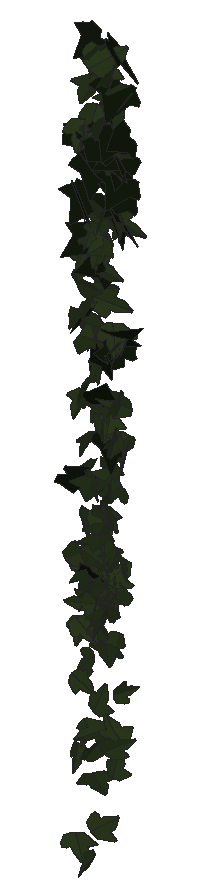
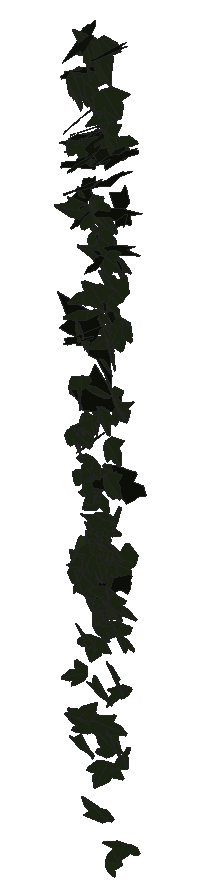
# SketchUp Ruby script. Lengths in inches.
U = 1.inch
M = Sketchup.active_model
def pt(a) = Geom::Point3d.new(a.map { |v| v * U })
def face(e, loops, mat)
  f = e.add_face(loops[0].map { |a| pt(a) })
  loops[1..].each { |l| e.add_face(l.map { |a| pt(a) }).erase! }
  f.material = f.back_material = mat if mat
  f
end
# faces: each face lists its corners as indices into pts; further lists are holes
def faces(e, pts, list, mat = nil) = list.each { |f| face(e, (f[0].is_a?(Array) ? f : [f]).map { |l| l.map { |i| pts[i] } }, mat) }
# xy, xz, yz: faces in a plane at the given z, y or x. An outline is a flat list of corners, or four numbers for a rectangle; further outlines are holes
def ring(l) = l.size == 4 ? [[l[0], l[1]], [l[2], l[1]], [l[2], l[3]], [l[0], l[3]]] : l.each_slice(2).to_a
def flat(e, list, mat, &to3) = list.each { |f| face(e, (f[0].is_a?(Array) ? f : [f]).map { |l| ring(l).map { |u, v| to3.(u, v) } }, mat) }
def xy(e, z, list, mat = nil) = flat(e, list, mat) { |x, y| [x, y, z] }
def xz(e, y, list, mat = nil) = flat(e, list, mat) { |x, z| [x, y, z] }
def yz(e, x, list, mat = nil) = flat(e, list, mat) { |y, z| [x, y, z] }
def lines(e, pts, list) = list.each { |a, b| e.add_line(pt(pts[a]), pt(pts[b])) }
# prism: a flat outline (further loops are holes) pulled along v
def prism(e, loops, v, mat = nil)
  f = face(e, loops, mat); d = Geom::Vector3d.new(v.map { |x| x * U })
  f.pushpull(f.normal.samedirection?(d) ? d.length : -d.length)
end
def box(e, o, s, mat = nil) = prism(e, [[o, [o[0] + s[0], o[1], o[2]], [o[0] + s[0], o[1] + s[1], o[2]], [o[0], o[1] + s[1], o[2]]]], [0, 0, s[2]], mat)
def at(x, y, z, deg = 0) = Geom::Transformation.translation(pt([x, y, z])) * Geom::Transformation.rotation(ORIGIN, Z_AXIS, deg.degrees)
def axes(o, x, y, z) = Geom::Transformation.new([*x, 0, *y, 0, *z, 0, *pt(o).to_a, 1])
def part(name) = M.definitions.add(name)
# library, detail: a bought-in or finely detailed component or shape, given as its bounding box
def library(name, o, s) = part(name).tap { |d| box(d.entities, o, s) }
def detail(e, o, s) = box(e.add_group.entities, o, s)
def put(e, d, t, mat = nil) = e.add_instance(d, t).tap { |i| i.material = mat if mat }
def group(e, t, mat = nil) = e.add_group.tap { |g| g.transformation = t; g.material = mat if mat }.entities
root = M.entities
M.materials.add("1026 AP 7946 SUNNY SIDE UP").color = [254, 231, 186]
M.materials.add("efeu1").color = [18, 25, 13]
M.materials.add("efeu2").color = [43, 57, 29]
c1 = part("ivyleaf_10")
p = [[0,0.5,-0.03],[-0.0625,2.02,-0.43],[-0.19,2.01,-0.46],[-0.54,1.05,-0.29],[-0.52,0.625,-0.18],[-0.83,0.76,-0.28],
  [-1.16,0.64,-0.33],[-1.15,0.33,-0.24],[-0.77,-0.39,0.02],[-0.3,-0.51,0.16],[0.04,-0.48,0.23],[-0.02,2.01,-0.4375],
  [-0.06,2.01,-0.43],[0.04,-0.49,0.23],[0.67,-0.49,0.14],[1.38,0.36,-0.2],[1.375,0.51,-0.24],[0.81,0.65,-0.19],
  [0.62,0.59,-0.15],[0.6,1.09,-0.28],[0.5,1.23,-0.31]]
faces(c1.entities,p,[[0,1,2,3,4,5,6,7,8,9,10],[11,12,0,13,14,15,16,17,18,19,20]],"efeu2")
c2 = part("ivyleaf_9")
p = [[1.54,2.16,1.25],[1.36,2.04,1.19],[-0.21,0.99,0.68],[-0.71,1.11,0.82],[-0.85,0.86,0.67],[-0.8,0.17,0.21],
  [-0.9,-0.01,0.1],[-0.67,-0.16,-0.02],[-0.08,-0.08,-0.05],[-0.03,-0.6,-0.4],[0.65,-0.88,-0.66],[0.83,-0.6,-0.49],
  [1.29,-0.42,-0.43],[1.8125,-0.07,-0.26],[1.21,0.44,0.15]]
faces(c2.entities,p,[[0,1,2,3,4,5,6,7,8,9,10,11,12,13,14]],"efeu1")
put(root,c1,axes([102.35,212.49,259.8],[-0.06688,-0.16371,0.15021],[0.07926,-0.15273,-0.16139],[0.33648,0.00344,0.06787]),"1026 AP 7946 SUNNY SIDE UP")
put(root,c2,axes([102.26,212.62,265.65],[-0.01705,-0.2455,-0.06618],[0.02244,0.06221,-0.25253],[0.39784,-0.01403,0.01141]),"1026 AP 7946 SUNNY SIDE UP")
put(root,c1,axes([102.35,212.43,261.7],[-0.06038,-0.19316,-0.16336],[0.10843,0.14488,-0.19955],[0.37656,-0.07269,0.03126]),"1026 AP 7946 SUNNY SIDE UP")
put(root,c1,axes([102.32,212.39,253.47],[0.05045,0.17084,0.12661],[0.05043,0.11791,-0.1782],[-0.32616,0.04466,-0.00797]),"1026 AP 7946 SUNNY SIDE UP")
put(root,c2,axes([102.45,212.63,264.3125],[-0.27752,-0.16463,0.01399],[0.00167,-0.02237,-0.24815],[0.25986,-0.17567,0.01654]),"1026 AP 7946 SUNNY SIDE UP")
put(root,c1,axes([102.34,212.45,254.69],[0.29099,-0.088,0.05389],[0.06145,-0.04027,-0.21044],[0.14922,0.18819,-0.01844]),"1026 AP 7946 SUNNY SIDE UP")
put(root,c1,axes([102.39,212.5,265.87],[0.29429,0.15936,-0.05989],[-0.04948,-0.05381,-0.25271],[-0.26261,0.18873,-0.0195]),"1026 AP 7946 SUNNY SIDE UP")
put(root,c1,axes([102.39,212.33,251.92],[0.03154,0.19338,-0.12033],[-0.03166,-0.11637,-0.20084],[-0.35472,0.02758,0.00722]),"1026 AP 7946 SUNNY SIDE UP")
put(root,c1,axes([102.47,212.65,258.25],[0.00646,-0.19667,0.0764],[-0.00698,-0.07536,-0.20301],[0.33105,0.00225,-0.00577]),"1026 AP 7946 SUNNY SIDE UP")
put(root,c1,axes([102.46,212.47,260.07],[0.11644,-0.22452,0.02799],[0.0032,-0.02926,-0.24361],[0.35584,0.07373,-0.00696]),"1026 AP 7946 SUNNY SIDE UP")
put(root,c1,axes([102.52,212.53,253.93],[0.18226,-0.16859,-0.09209],[-0.09963,0.06347,-0.20983],[0.28228,0.13125,-0.0146]),"1026 AP 7946 SUNNY SIDE UP")
put(root,c1,axes([102.54,212.65,266.89],[-0.18408,-0.19871,0.10836],[-0.03233,-0.10989,-0.23556],[0.35289,-0.11373,0.03495]),"1026 AP 7946 SUNNY SIDE UP")
put(root,c1,axes([102.47,212.64,263.22],[-0.01801,-0.16096,0.17874],[0.05034,-0.17407,-0.16434],[0.36977,0.01586,0.03108]),"1026 AP 7946 SUNNY SIDE UP")
put(root,c2,axes([102.58,212.61,263.4],[-0.28153,-0.13286,0.10644],[-0.101,-0.08667,-0.22833],[0.24541,-0.18809,0.02814]),"1026 AP 7946 SUNNY SIDE UP")
put(root,c1,axes([102.35,212.23,256.3],[-0.06701,-0.08618,0.22956],[0.11622,0.21101,0.09965],[-0.358,0.08463,-0.01062]),"1026 AP 7946 SUNNY SIDE UP")
put(root,c1,axes([102.36,212.31,249.9],[0.27831,0.09746,0.05304],[0.08373,0.00848,-0.2073],[-0.15129,0.18398,-0.01716]),"1026 AP 7946 SUNNY SIDE UP")
put(root,c1,axes([102.49,212.57,255.39],[0.04011,-0.18599,0.09118],[0.01307,-0.08925,-0.19389],[0.32434,0.02659,-0.00347]),"1026 AP 7946 SUNNY SIDE UP")
put(root,c1,axes([102.6875,212.34,255.31],[0.14234,-0.04484,-0.19724],[-0.29436,0.04394,-0.10166],[0.09334,0.20694,-0.01983]),"1026 AP 7946 SUNNY SIDE UP")
put(root,c2,axes([102.27,212.21,258.11],[0.06747,0.06336,-0.23946],[0.13637,0.2166,0.07846],[0.35401,-0.09551,0.01541]),"1026 AP 7946 SUNNY SIDE UP")
put(root,c1,axes([102.45,212.4,261.6875],[-0.35605,0.04412,-0.08694],[0.11989,-0.04748,-0.23591],[-0.09028,-0.23703,0.02958]),"1026 AP 7946 SUNNY SIDE UP")
put(root,c1,axes([102.47,212.54,252.38],[0.2449,-0.13207,0.04891],[0.04208,-0.04281,-0.21006],[0.21704,0.15732,-0.01446]),"1026 AP 7946 SUNNY SIDE UP")
put(root,c1,axes([102.55,212.52,258.95],[-0.00492,-0.21341,0.06721],[-0.00372,-0.06642,-0.22026],[0.35144,-0.00369,-0.00139]),"1026 AP 7946 SUNNY SIDE UP")
put(root,c1,axes([102.56,212.54,261.24],[0.15576,-0.20161,-0.06929],[-0.03045,0.06407,-0.23078],[0.33222,0.10039,0.01133]),"1026 AP 7946 SUNNY SIDE UP")
put(root,c2,axes([102.28,212.41,264.36],[0.12024,-0.04405,-0.26678],[0.38522,-0.08463,0.08895],[-0.14795,-0.25616,0.01478]),"1026 AP 7946 SUNNY SIDE UP")
put(root,c1,axes([102.54,212.54,265.95],[0.05317,-0.21396,0.12699],[0.05774,-0.11992,-0.2233],[0.38492,0.04754,0.01595]),"1026 AP 7946 SUNNY SIDE UP")
put(root,c2,axes([102.6,212.73,267.83],[-0.17957,-0.15955,0.17401],[-0.09036,-0.16399,-0.1995],[0.35507,-0.12242,0.03723]),"1026 AP 7946 SUNNY SIDE UP")
put(root,c1,axes([102.57,212.34,255.96],[-0.13561,-0.18494,-0.07859],[0.06627,0.06325,-0.20956],[0.30687,-0.09538,0.01052]),"1026 AP 7946 SUNNY SIDE UP")
put(root,c1,axes([102.59,212.23,257.28],[-0.12845,0.21034,0.04155],[-0.04464,0.03087,-0.23176],[-0.33345,-0.08516,0.01502]),"1026 AP 7946 SUNNY SIDE UP")
put(root,c2,axes([102.47,212.33,256.03],[0.3726,-0.00112,-0.04759],[-0.07253,-0.01936,-0.24343],[-0.00409,0.24065,-0.01839]),"1026 AP 7946 SUNNY SIDE UP")
put(root,c2,axes([102.52,212.63,265.01],[-0.08696,-0.24295,0.04112],[-0.00248,-0.04197,-0.25681],[0.38749,-0.05479,0.00758]),"1026 AP 7946 SUNNY SIDE UP")
put(root,c2,axes([102.4,212.68,265.61],[0.07405,-0.2329,0.07996],[0.11217,-0.06398,-0.23868],[0.37005,0.066,0.05635]),"1026 AP 7946 SUNNY SIDE UP")
put(root,c1,axes([102.45,212.42,256.2],[0.27207,0.08357,0.10736],[0.15556,0.03328,-0.1974],[-0.14028,0.19898,-0.01068]),"1026 AP 7946 SUNNY SIDE UP")
put(root,c1,axes([102.59,212.45,262],[0.06884,-0.19635,0.12936],[0.07423,-0.11879,-0.20719],[0.35985,0.06207,0.01799]),"1026 AP 7946 SUNNY SIDE UP")
put(root,c1,axes([102.62,212.63,263.62],[0.00223,-0.16796,0.17498],[0.05261,-0.169,-0.17248],[0.37298,0.02484,0.02328]),"1026 AP 7946 SUNNY SIDE UP")
put(root,c1,axes([102.48,212.29,254.8],[0.17054,0.15089,0.11318],[0.12211,0.07798,-0.19035],[-0.26601,0.13254,-0.01482]),"1026 AP 7946 SUNNY SIDE UP")
put(root,c1,axes([102.58,212.34,263.12],[0.34807,-0.11427,0.03463],[0.03134,-0.03578,-0.2558],[0.18495,0.22112,-0.02182]),"1026 AP 7946 SUNNY SIDE UP")
put(root,c2,axes([102.7,212.41,262.04],[-0.24468,0.12053,-0.15406],[0.16687,-0.10751,-0.20274],[-0.25273,-0.18768,0.01529]),"1026 AP 7946 SUNNY SIDE UP")
put(root,c1,axes([102.63,212.49,256.29],[-0.28041,0.1082,-0.01109],[0.00081,-0.02101,-0.21424],[-0.17107,-0.17745,0.01717]),"1026 AP 7946 SUNNY SIDE UP")
put(root,c1,axes([102.55,212.55,255.59],[-0.31334,0.01739,-0.10443],[0.15408,-0.03577,-0.20477],[-0.04965,-0.22074,0.02362]),"1026 AP 7946 SUNNY SIDE UP")
put(root,c1,axes([102.9,212.38,256.55],[-0.04006,0.02041,0.21325],[-0.32556,0.01627,-0.02783],[-0.02942,-0.20781,0.01753]),"1026 AP 7946 SUNNY SIDE UP")
put(root,c1,axes([102.63,212.42,249.5],[0.04049,-0.09162,0.19518],[0.08019,-0.18301,-0.09911],[0.32181,0.05713,0.00014]),"1026 AP 7946 SUNNY SIDE UP")
put(root,c1,axes([102.43,212.37,262.37],[-0.16155,-0.01511,0.23225],[0.34997,-0.05,0.10071],[0.06203,0.24274,0.03669]),"1026 AP 7946 SUNNY SIDE UP")
put(root,c1,axes([102.71,212.64,267.55],[0.05943,-0.24383,0.09258],[0.0274,-0.08964,-0.2547],[0.40846,0.04149,0.00362]),"1026 AP 7946 SUNNY SIDE UP")
put(root,c1,axes([102.93,212.44,255.43],[-0.1324,0.03818,0.19554],[-0.29904,0.02125,-0.0913],[-0.05529,-0.20636,0.02552]),"1026 AP 7946 SUNNY SIDE UP")
put(root,c1,axes([102.7,212.49,266.33],[0.19476,0.19756,-0.1056],[-0.07438,-0.09257,-0.2406],[-0.3428,0.13233,-0.00779]),"1026 AP 7946 SUNNY SIDE UP")
put(root,c1,axes([102.73,212.5,261.55],[0.22706,-0.18245,-0.0064],[-0.01865,-0.00279,-0.23945],[0.28639,0.14447,-0.01051]),"1026 AP 7946 SUNNY SIDE UP")
put(root,c1,axes([102.79,212.28,258.09],[-0.26168,-0.14278,0.04479],[-0.0326,-0.04359,-0.22528],[0.23278,-0.16661,0.0188]),"1026 AP 7946 SUNNY SIDE UP")
put(root,c1,axes([102.64,212.33,258.17],[-0.20732,0.14816,-0.12167],[0.10827,-0.09767,-0.20455],[-0.27845,-0.1483,0.01106]),"1026 AP 7946 SUNNY SIDE UP")
put(root,c1,axes([102.76,212.55,259.66],[0.29039,-0.09391,-0.06018],[-0.05984,0.05171,-0.21121],[0.16281,0.1865,0.02971]),"1026 AP 7946 SUNNY SIDE UP")
put(root,c1,axes([102.96,212.39,264.07],[0.12849,-0.04564,-0.24083],[-0.26672,0.16197,-0.09281],[0.26236,0.18701,0.02359]),"1026 AP 7946 SUNNY SIDE UP")
put(root,c1,axes([102.63,212.26,261.34],[-0.09141,-0.13054,-0.22985],[0.23572,0.16836,-0.14121],[0.32989,-0.15647,0.03721]),"1026 AP 7946 SUNNY SIDE UP")
put(root,c1,axes([102.96,212.38,254.7],[-0.14109,0.04893,-0.18486],[-0.21403,0.11895,0.10407],[0.19992,0.16187,-0.01905]),"1026 AP 7946 SUNNY SIDE UP")
put(root,c1,axes([102.81,212.4,260.63],[0.20946,-0.16127,-0.07361],[-0.0465,0.0667,-0.21424],[0.27285,0.13517,0.02]),"1026 AP 7946 SUNNY SIDE UP")
put(root,c1,axes([102.82,212.57,256.3],[-0.11438,-0.19764,0.01536],[0.00226,-0.0176,-0.21693],[0.31178,-0.07238,0.00721]),"1026 AP 7946 SUNNY SIDE UP")
put(root,c1,axes([102.93,212.39,252.5],[-0.11208,-0.06206,0.20843],[-0.15492,-0.17963,-0.09341],[0.2951,-0.11787,0.03013]),"1026 AP 7946 SUNNY SIDE UP")
put(root,c2,axes([102.71,212.3,262.97],[-0.19435,0.16444,0.14503],[0.10837,-0.12265,0.21061],[0.32165,0.14068,0.01667]),"1026 AP 7946 SUNNY SIDE UP")
put(root,c1,axes([102.86,212.62,262.35],[-0.1773,-0.17051,0.09972],[-0.03045,-0.10253,-0.20782],[0.30756,-0.10845,0.03691]),"1026 AP 7946 SUNNY SIDE UP")
put(root,c1,axes([102.85,212.4375,267.8],[-0.00621,-0.27152,0.04252],[-0.00149,-0.04281,-0.28],[0.43221,-0.00405,-0.00035]),"1026 AP 7946 SUNNY SIDE UP")
put(root,c1,axes([102.76,212.24,251.94],[-0.03776,-0.18434,0.11022],[0.01821,0.10743,0.19213],[-0.33547,0.02658,-0.00198]),"1026 AP 7946 SUNNY SIDE UP")
put(root,c2,axes([102.96,212.33,261.01],[0.18081,-0.01456,-0.22662],[-0.3465,-0.00994,-0.11809],[-0.00327,0.24794,-0.01659]),"1026 AP 7946 SUNNY SIDE UP")
put(root,c1,axes([102.74,212.44,255.36],[0.15674,-0.11924,0.15997],[0.13769,-0.12954,-0.16045],[0.27628,0.13221,-0.01079]),"1026 AP 7946 SUNNY SIDE UP")
put(root,c1,axes([102.65,212.32,256.42],[-0.10361,0.00924,-0.2087],[0.28233,-0.09647,-0.06525],[-0.14839,-0.18999,0.02158]),"1026 AP 7946 SUNNY SIDE UP")
put(root,c2,axes([102.69,212.67,265.78],[0.15407,-0.22625,0.04418],[0.00857,-0.04571,-0.25392],[0.36238,0.09727,-0.01278]),"1026 AP 7946 SUNNY SIDE UP")
put(root,c1,axes([102.73,212.56,257.21],[0.26402,0.08567,0.09557],[0.14179,0.02554,-0.19331],[-0.13819,0.18989,-0.01576]),"1026 AP 7946 SUNNY SIDE UP")
put(root,c1,axes([102.9375,212.34,256.85],[-0.20049,-0.17309,0.01224],[0.00497,-0.01828,-0.22115],[0.27287,-0.12684,0.01302]),"1026 AP 7946 SUNNY SIDE UP")
put(root,c2,axes([102.91,212.5,262.97],[0.07562,-0.16893,-0.2053],[0.10457,-0.18703,0.17965],[-0.39607,-0.08163,0.00824]),"1026 AP 7946 SUNNY SIDE UP")
put(root,c1,axes([102.87,212.27,251.49],[-0.2415,-0.14023,-0.07938],[0.10572,0.03915,-0.21343],[0.22764,-0.16695,0.01491]),"1026 AP 7946 SUNNY SIDE UP")
put(root,c1,axes([102.96,212.38,257.1],[-0.15107,-0.18973,0.03619],[-0.01104,-0.03698,-0.21905],[0.30352,-0.09578,0.01005]),"1026 AP 7946 SUNNY SIDE UP")
put(root,c1,axes([102.97,212.29,259.34],[0.03294,0.06602,-0.22814],[-0.03486,0.22229,0.06729],[0.36225,0.01539,0.02722]),"1026 AP 7946 SUNNY SIDE UP")
put(root,c1,axes([102.99,212.58,258.19],[-0.14859,-0.1483,0.11618],[-0.02748,-0.11975,-0.1767],[0.29247,-0.0866,0.04242]),"1026 AP 7946 SUNNY SIDE UP")
put(root,c1,axes([102.95,212.72,257.84],[-0.02867,-0.01884,-0.22602],[-0.08503,-0.21291,0.02223],[-0.33548,0.05558,0.01368]),"1026 AP 7946 SUNNY SIDE UP")
put(root,c2,axes([102.82,212.49,259.8],[0.36817,0.00914,0.07023],[-0.10803,0.02458,0.24003],[0.00292,-0.24261,0.02553]),"1026 AP 7946 SUNNY SIDE UP")
put(root,c1,axes([102.98,212.36,255.01],[0.00994,-0.19641,0.07408],[0.00485,-0.07296,-0.20287],[0.32945,0.007,0.00075]),"1026 AP 7946 SUNNY SIDE UP")
put(root,c1,axes([102.93,212.51,256.47],[-0.2244,-0.13976,-0.08974],[0.11093,0.05111,-0.20512],[0.23326,-0.15876,0.01122]),"1026 AP 7946 SUNNY SIDE UP")
put(root,c1,axes([102.75,212.47,256.36],[0.22526,-0.03542,0.18997],[0.27305,-0.06393,-0.15184],[0.11317,0.22476,-0.0118]),"1026 AP 7946 SUNNY SIDE UP")
put(root,c1,axes([102.97,212.49,264.2],[0.08634,-0.22125,0.085],[0.03789,-0.08032,-0.23528],[0.37006,0.05984,0.00426]),"1026 AP 7946 SUNNY SIDE UP")
put(root,c1,axes([103,212.46,254.36],[-0.31861,-0.00816,-0.00457],[0.00812,-0.01967,-0.20803],[0.0121,-0.20172,0.01928]),"1026 AP 7946 SUNNY SIDE UP")
put(root,c1,axes([103.03,212.28,266.32],[0.00372,-0.2545,-0.00986],[-0.00238,0.00811,-0.26215],[0.40038,0.00241,-0.00147]),"1026 AP 7946 SUNNY SIDE UP")
put(root,c1,axes([102.95,212.32,263.54],[0.3659,-0.09857,0.02796],[0.0261,-0.03156,-0.2595],[0.15887,0.23221,-0.02178]),"1026 AP 7946 SUNNY SIDE UP")
put(root,c1,axes([102.91,212.28,253.09],[0.31639,-0.11508,-0.0092],[0.03091,0.01779,0.23749],[-0.17877,-0.2006,0.02478]),"1026 AP 7946 SUNNY SIDE UP")
put(root,c1,axes([102.96,212.59,259.42],[0.14351,0.18442,-0.07003],[-0.0312,-0.06708,-0.21205],[-0.30805,0.09271,-0.01115]),"1026 AP 7946 SUNNY SIDE UP")
put(root,c1,axes([103.02,212.6875,255.87],[-0.0734,-0.14735,0.13619],[0.02565,-0.13905,-0.15358],[0.3111,-0.0233,0.04479]),"1026 AP 7946 SUNNY SIDE UP")
put(root,c1,axes([103.05,212.27,255.25],[-0.0927,-0.20328,0.02192],[-0.00115,-0.02314,-0.2181],[0.32157,-0.05868,0.00554]),"1026 AP 7946 SUNNY SIDE UP")
put(root,c1,axes([103.02,212.42,263.49],[-0.1103,0.00084,0.23742],[0.04904,-0.23865,0.00928],[0.35904,0.03286,0.07167]),"1026 AP 7946 SUNNY SIDE UP")
put(root,c1,axes([102.95,212.54,256.34],[-0.30799,0.06069,0.09521],[0.14679,-0.00865,0.21042],[0.09231,0.21626,-0.01694]),"1026 AP 7946 SUNNY SIDE UP")
put(root,c1,axes([102.98,212.57,258.4375],[-0.27494,0.08473,-0.0655],[0.07334,-0.04962,-0.19904],[-0.15007,-0.17949,0.02274]),"1026 AP 7946 SUNNY SIDE UP")
put(root,c1,axes([103.01,212.375,255.98],[-0.10776,-0.16622,-0.11787],[0.09152,0.09838,-0.1841],[0.30293,-0.08885,0.01369]),"1026 AP 7946 SUNNY SIDE UP")
put(root,c2,axes([102.95,212.6,258.9375],[-0.0074,-0.23208,0.08216],[0.00786,-0.08115,-0.23952],[0.38646,-0.00279,0.00644]),"1026 AP 7946 SUNNY SIDE UP")
put(root,c1,axes([103.09,212.38,257.88],[-0.00362,-0.16695,-0.14693],[0.0192,0.14137,-0.17099],[0.34377,-0.00965,0.008]),"1026 AP 7946 SUNNY SIDE UP")
put(root,c1,axes([102.98,212.44,255.5],[-0.2139,-0.12526,0.12514],[0.13079,0.08987,0.19085],[-0.24207,0.15924,-0.00747]),"1026 AP 7946 SUNNY SIDE UP")
put(root,c1,axes([102.91,212.41,262.1875],[0.07956,0.08284,0.23693],[0.18359,0.1976,-0.09883],[-0.3369,0.12724,0.00209]),"1026 AP 7946 SUNNY SIDE UP")
put(root,c1,axes([103,212.46,255.18],[-0.26004,0.09458,0.12748],[0.18206,-0.0449,0.19535],[0.1628,0.20128,-0.01483]),"1026 AP 7946 SUNNY SIDE UP")
put(root,c1,axes([102.82,212.3,263.02],[-0.0721,-0.02223,-0.25611],[0.36068,-0.10309,-0.03471],[-0.15424,-0.23069,0.03856]),"1026 AP 7946 SUNNY SIDE UP")
put(root,c1,axes([103.4,212.47,259.95],[-0.0056,-0.00501,-0.24248],[-0.36762,0.02749,0.0032],[0.04311,0.23376,-0.00419]),"1026 AP 7946 SUNNY SIDE UP")
put(root,c1,axes([103.04,212.32,257.53],[-0.28512,0.01924,-0.09452],[0.1358,-0.04402,-0.18538],[-0.05777,-0.19844,0.03073]),"1026 AP 7946 SUNNY SIDE UP")
put(root,c1,axes([103.29,212.5,258.02],[-0.23782,0.0635,0.12449],[-0.20686,-0.02156,-0.15856],[-0.05538,-0.19216,0.05766]),"1026 AP 7946 SUNNY SIDE UP")
put(root,c2,axes([103.07,212.6,265.93],[-0.15687,-0.21124,0.09586],[0.01567,-0.10647,-0.2356],[0.36338,-0.0866,0.05154]),"1026 AP 7946 SUNNY SIDE UP")
put(root,c1,axes([103.32,212.41,266.65],[0.13078,-0.1078,-0.24083],[-0.24917,0.17135,-0.13885],[0.31789,0.17866,-0.00976]),"1026 AP 7946 SUNNY SIDE UP")
put(root,c1,axes([103.05,212.39,255.96],[-0.07647,0.15862,-0.14523],[0.05629,-0.13736,-0.17166],[-0.32986,-0.06021,0.00437]),"1026 AP 7946 SUNNY SIDE UP")
put(root,c1,axes([102.93,212.26,250.35],[0.26486,-0.04068,-0.1407],[0.22,0.00897,0.17537],[-0.04065,-0.21652,0.03239]),"1026 AP 7946 SUNNY SIDE UP")
put(root,c1,axes([103.21,212.3,256.71],[0.23492,-0.18287,-0.07524],[-0.09293,0.04444,-0.24239],[0.29472,0.15978,-0.01646]),"1026 AP 7946 SUNNY SIDE UP")
put(root,c1,axes([103.36,212.28,255.45],[-0.07085,0.03551,0.20194],[-0.29857,0.05244,-0.0545],[-0.09369,-0.19397,0.02097]),"1026 AP 7946 SUNNY SIDE UP")
put(root,c1,axes([103.27,212.23,256.49],[-0.00274,0.01561,0.22521],[-0.2132,0.17157,-0.01274],[-0.27058,-0.13535,0.00775]),"1026 AP 7946 SUNNY SIDE UP")
put(root,c1,axes([103.21,212.28,264.2],[0.13805,-0.18834,-0.1416],[-0.03262,0.13886,-0.21049],[0.36419,0.08383,0.03482]),"1026 AP 7946 SUNNY SIDE UP")
put(root,c2,axes([102.98,212.3,265.78],[0.05409,-0.21683,-0.12861],[0.06565,0.12802,-0.21863],[0.38692,0.00859,0.05507]),"1026 AP 7946 SUNNY SIDE UP")
put(root,c1,axes([103.4,212.42,255.78],[-0.22896,-0.00376,0.17647],[-0.25813,-0.0614,-0.14549],[0.07726,-0.21629,0.03686]),"1026 AP 7946 SUNNY SIDE UP")
put(root,c1,axes([103.16,212.25,257.64],[-0.23608,0.13322,-0.0325],[0.02061,-0.03374,-0.2063],[-0.21456,-0.14982,0.01595]),"1026 AP 7946 SUNNY SIDE UP")
put(root,c2,axes([103.36,212.52,261.02],[-0.27129,-0.17323,0.05468],[0.04571,0.04725,0.25183],[-0.28167,0.17452,-0.0118]),"1026 AP 7946 SUNNY SIDE UP")
put(root,c1,axes([103.12,212.63,254.54],[0.2695,-0.1066,0.07618],[0.08363,-0.05511,-0.20747],[0.18666,0.1786,-0.01703]),"1026 AP 7946 SUNNY SIDE UP")
put(root,c1,axes([102.94,212.23,267.6],[0.32317,0.02905,-0.21488],[0.3031,0.09199,0.20924],[0.134,-0.27812,0.04494]),"1026 AP 7946 SUNNY SIDE UP")
put(root,c1,axes([103.03,212.56,256.09],[0.02245,-0.01598,0.21388],[0.24487,-0.13745,-0.02273],[0.21754,0.15637,0.00351]),"1026 AP 7946 SUNNY SIDE UP")
put(root,c1,axes([103.27,212.45,266.9],[-0.19379,-0.21549,0.06983],[-0.00926,-0.0755,-0.25415],[0.35566,-0.11938,0.03143]),"1026 AP 7946 SUNNY SIDE UP")
put(root,c2,axes([103.12,212.72,265.2],[-0.05746,-0.19918,0.14667],[0.00337,-0.14534,-0.2081],[0.38599,-0.02838,0.02365]),"1026 AP 7946 SUNNY SIDE UP")
put(root,c1,axes([103.26,212.27,267.5],[-0.00652,-0.25068,-0.09443],[0.00073,0.09024,-0.25776],[0.41893,-0.00406,-0.00102]),"1026 AP 7946 SUNNY SIDE UP")
put(root,c1,axes([103.3,212.67,259.07],[-0.14002,-0.14341,0.13664],[-0.042,-0.13633,-0.1701],[0.30515,-0.08457,0.03929]),"1026 AP 7946 SUNNY SIDE UP")
put(root,c2,axes([103.1,212.67,263.99],[0.04913,-0.20168,0.13455],[0.01484,-0.13173,-0.21081],[0.37851,0.03134,-0.0092]),"1026 AP 7946 SUNNY SIDE UP")
put(root,c2,axes([103.26,212.6875,264.5625],[-0.18319,-0.17756,0.12429],[-0.04707,-0.12362,-0.21614],[0.33515,-0.11441,0.03757]),"1026 AP 7946 SUNNY SIDE UP")
put(root,c2,axes([103.13,212.73,265.7],[-0.00963,-0.23467,0.08562],[0.01171,-0.0846,-0.24215],[0.39198,-0.00324,0.00934]),"1026 AP 7946 SUNNY SIDE UP")
put(root,c1,axes([103.29,212.39,259.2],[0.0373,-0.22202,0.02118],[-0.00027,-0.02196,-0.23014],[0.35079,0.02359,-0.00243]),"1026 AP 7946 SUNNY SIDE UP")
put(root,c1,axes([103.35,212.45,265.5],[-0.23377,-0.18557,0.08689],[-0.03473,-0.0904,-0.2425],[0.31932,-0.14568,0.03724]),"1026 AP 7946 SUNNY SIDE UP")
put(root,c2,axes([103.11,212.48,267.99],[0.3,-0.18078,-0.10911],[-0.12468,0.06879,-0.27034],[0.30408,0.20657,-0.00319]),"1026 AP 7946 SUNNY SIDE UP")
put(root,c1,axes([103.28,212.6,255.71],[0.03518,0.0856,-0.18947],[-0.05996,-0.18046,-0.09212],[-0.314,0.04405,-0.00364]),"1026 AP 7946 SUNNY SIDE UP")
put(root,c1,axes([103.36,212.37,252.53],[0.21103,0.13751,0.07109],[-0.09128,-0.03843,0.1972],[0.22344,-0.14557,0.01343]),"1026 AP 7946 SUNNY SIDE UP")
put(root,c1,axes([103.33,212.48,261.31],[0.02884,-0.22224,0.01555],[-0.00287,-0.01656,-0.2298],[0.35038,0.01816,-0.00316]),"1026 AP 7946 SUNNY SIDE UP")
put(root,c1,axes([103.23,212.39,261.625],[0.24175,0.19957,-0.00558],[0.01207,-0.01417,-0.25917],[-0.31373,0.15323,-0.01427]),"1026 AP 7946 SUNNY SIDE UP")
put(root,c1,axes([103.32,212.4,260.05],[0.01596,-0.22782,-0.10483],[0.04013,0.10097,-0.23264],[0.38945,-0.00107,0.02827]),"1026 AP 7946 SUNNY SIDE UP")
put(root,c1,axes([103.28,212.44,259.24],[-0.00239,0.13774,-0.19572],[-0.00746,-0.19075,-0.14296],[-0.3699,0.00296,0.00415]),"1026 AP 7946 SUNNY SIDE UP")
put(root,c1,axes([103.37,212.58,266.99],[-0.06609,-0.23288,0.11592],[0.01157,-0.11635,-0.24309],[0.40743,-0.03447,0.0257]),"1026 AP 7946 SUNNY SIDE UP")
put(root,c2,axes([103.45,212.57,265.57],[-0.25593,-0.11772,0.15066],[-0.12968,-0.12999,-0.2022],[0.26609,-0.17657,0.04636]),"1026 AP 7946 SUNNY SIDE UP")
put(root,c2,axes([103.33,212.48,267.1],[-0.2227,-0.22101,0.01495],[0.00309,-0.01996,-0.27024],[0.34839,-0.1411,0.01195]),"1026 AP 7946 SUNNY SIDE UP")
put(root,c1,axes([103.37,212.51,261.4],[0.181,-0.19419,-0.03854],[-0.02225,0.03381,-0.2323],[0.30984,0.11587,0.00583]),"1026 AP 7946 SUNNY SIDE UP")
put(root,c1,axes([103.21,212.39,256.02],[0.25085,0.05623,-0.13294],[0.16259,0.08622,0.17048],[0.15086,-0.18642,0.03732]),"1026 AP 7946 SUNNY SIDE UP")
put(root,c2,axes([103.13,212.42,261.375],[0.32685,0.1304,-0.02957],[0.02159,0.03332,0.25208],[0.20908,-0.20728,0.02019]),"1026 AP 7946 SUNNY SIDE UP")
put(root,c1,axes([103.34,212.31,251.74],[0.30599,-0.07678,0.02667],[-0.02226,0.03521,0.21388],[-0.12567,-0.19319,0.02703]),"1026 AP 7946 SUNNY SIDE UP")
put(root,c2,axes([103.4,212.63,265.93],[-0.12925,-0.12394,0.21377],[-0.09155,-0.20332,-0.14955],[0.36984,-0.09364,0.03769]),"1026 AP 7946 SUNNY SIDE UP")
put(root,c2,axes([103.21,212.38,264.39],[0.26933,-0.18603,-0.01789],[-0.03778,0,-0.25988],[0.2912,0.17206,-0.01717]),"1026 AP 7946 SUNNY SIDE UP")
put(root,c2,axes([103.43,212.48,265.04],[-0.22031,-0.19615,0.0544],[-0.02458,-0.05489,-0.2479],[0.31892,-0.13973,0.01847]),"1026 AP 7946 SUNNY SIDE UP")
put(root,c1,axes([103.14,212.58,264.04],[-0.12013,0.00417,-0.24514],[0.35862,-0.0702,-0.07711],[-0.10704,-0.23988,0.01678]),"1026 AP 7946 SUNNY SIDE UP")
put(root,c1,axes([103.45,212.58,266.84],[0.094,-0.25328,0.00808],[-0.0061,-0.01045,-0.26808],[0.39847,0.05959,-0.00601]),"1026 AP 7946 SUNNY SIDE UP")
put(root,c1,axes([103.46,212.3,264.17],[0.21472,-0.19397,-0.07861],[-0.04099,0.0733,-0.24308],[0.32454,0.13759,0.02131]),"1026 AP 7946 SUNNY SIDE UP")
put(root,c1,axes([103.33,212.625,258.82],[0.1584,-0.12416,0.14779],[0.12572,-0.1204,-0.16508],[0.27147,0.1282,-0.00979]),"1026 AP 7946 SUNNY SIDE UP")
put(root,c1,axes([103.43,212.41,256.41],[0.15989,-0.08203,-0.19334],[0.00361,0.20954,-0.09207],[0.32136,0.03846,0.09723]),"1026 AP 7946 SUNNY SIDE UP")
put(root,c1,axes([103.38,212.4,253.47],[0.01606,-0.03074,0.20578],[0.01228,0.20009,0.03245],[-0.31782,0.00618,0.01165]),"1026 AP 7946 SUNNY SIDE UP")
put(root,c1,axes([103.3125,212.21,252.26],[-0.10606,-0.10917,0.18167],[0.12121,0.15965,0.13266],[-0.30364,0.10186,-0.01049]),"1026 AP 7946 SUNNY SIDE UP")
